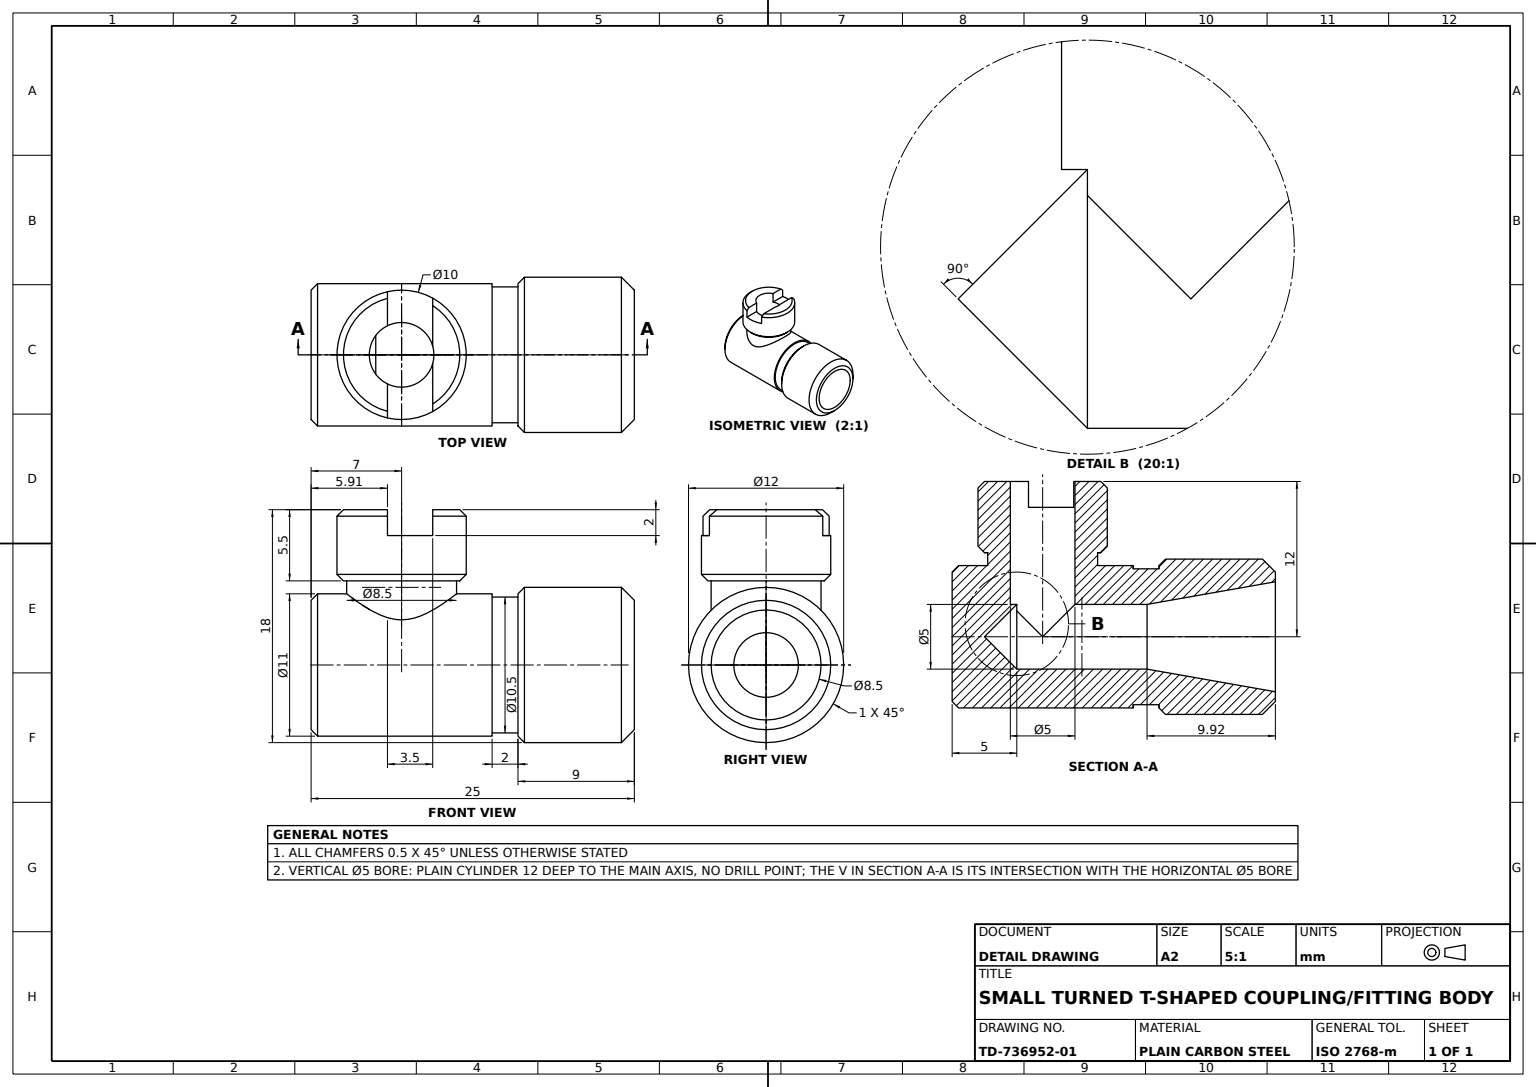
ISO-10303-21;
HEADER;
FILE_DESCRIPTION((''),'2;1');
FILE_NAME('','',(''),(''),'','','');
FILE_SCHEMA(('AUTOMOTIVE_DESIGN'));
ENDSEC;
DATA;
#1=APPLICATION_CONTEXT('');
#2=PRODUCT_CONTEXT('',#1,'mechanical');
#3=PRODUCT('','','',(#2));
#4=PRODUCT_DEFINITION_FORMATION('','',#3);
#5=PRODUCT_DEFINITION_CONTEXT('',#1,'design');
#6=PRODUCT_DEFINITION('','',#4,#5);
#7=PRODUCT_DEFINITION_SHAPE('','',#6);
#8=(LENGTH_UNIT()NAMED_UNIT(*)SI_UNIT(.MILLI.,.METRE.));
#9=(NAMED_UNIT(*)PLANE_ANGLE_UNIT()SI_UNIT($,.RADIAN.));
#10=(NAMED_UNIT(*)SI_UNIT($,.STERADIAN.)SOLID_ANGLE_UNIT());
#11=UNCERTAINTY_MEASURE_WITH_UNIT(LENGTH_MEASURE(1.E-05),#8,'distance_accuracy_value','');
#12=(GEOMETRIC_REPRESENTATION_CONTEXT(3)GLOBAL_UNCERTAINTY_ASSIGNED_CONTEXT((#11))GLOBAL_UNIT_ASSIGNED_CONTEXT((#8,#9,#10))REPRESENTATION_CONTEXT('',''));
#13=CARTESIAN_POINT('',(16.5,0.,6.));
#14=VERTEX_POINT('',#13);
#15=CARTESIAN_POINT('',(16.5,0.,-6.));
#16=VERTEX_POINT('',#15);
#17=CARTESIAN_POINT('',(16.5,0.,0.));
#18=DIRECTION('',(1.,0.,0.));
#19=DIRECTION('',(0.,0.,-1.));
#20=AXIS2_PLACEMENT_3D('',#17,#18,#19);
#21=CIRCLE('',#20,6.);
#22=EDGE_CURVE('',#14,#16,#21,.T.);
#23=ORIENTED_EDGE('',*,*,#22,.T.);
#24=CARTESIAN_POINT('',(24.,0.,-6.));
#25=VERTEX_POINT('',#24);
#26=CARTESIAN_POINT('',(-29.985577,0.,-6.));
#27=DIRECTION('',(-1.,0.,0.));
#28=VECTOR('',#27,1000.);
#29=LINE('',#26,#28);
#30=EDGE_CURVE('',#25,#16,#29,.T.);
#31=ORIENTED_EDGE('',*,*,#30,.F.);
#32=CARTESIAN_POINT('',(24.,0.,6.));
#33=VERTEX_POINT('',#32);
#34=CARTESIAN_POINT('',(24.,0.,0.));
#35=DIRECTION('',(0.,0.,1.));
#36=AXIS2_PLACEMENT_3D('',#34,#27,#35);
#37=CIRCLE('',#36,6.);
#38=EDGE_CURVE('',#25,#33,#37,.T.);
#39=ORIENTED_EDGE('',*,*,#38,.T.);
#40=CARTESIAN_POINT('',(-29.985577,0.,6.));
#41=LINE('',#40,#28);
#42=EDGE_CURVE('',#33,#14,#41,.T.);
#43=ORIENTED_EDGE('',*,*,#42,.T.);
#44=EDGE_LOOP('',(#23,#31,#39,#43));
#45=FACE_OUTER_BOUND('',#44,.T.);
#46=CARTESIAN_POINT('',(-29.985577,0.,0.));
#47=AXIS2_PLACEMENT_3D('',#46,#27,#35);
#48=CYLINDRICAL_SURFACE('',#47,6.);
#49=ADVANCED_FACE('',(#45),#48,.T.);
#50=CARTESIAN_POINT('',(16.,0.,-5.5));
#51=VERTEX_POINT('',#50);
#52=DIRECTION('',(0.707106781,0.,-0.707106781));
#53=VECTOR('',#52,1000.);
#54=LINE('',#50,#53);
#55=EDGE_CURVE('',#51,#16,#54,.T.);
#56=ORIENTED_EDGE('',*,*,#55,.T.);
#57=ORIENTED_EDGE('',*,*,#22,.F.);
#58=CARTESIAN_POINT('',(16.,0.,5.5));
#59=VERTEX_POINT('',#58);
#60=DIRECTION('',(0.707106781,0.,0.707106781));
#61=VECTOR('',#60,1000.);
#62=LINE('',#58,#61);
#63=EDGE_CURVE('',#59,#14,#62,.T.);
#64=ORIENTED_EDGE('',*,*,#63,.F.);
#65=CARTESIAN_POINT('',(16.,0.,0.));
#66=AXIS2_PLACEMENT_3D('',#65,#27,#19);
#67=CIRCLE('',#66,5.5);
#68=EDGE_CURVE('',#51,#59,#67,.T.);
#69=ORIENTED_EDGE('',*,*,#68,.F.);
#70=EDGE_LOOP('',(#56,#57,#64,#69));
#71=FACE_OUTER_BOUND('',#70,.T.);
#72=AXIS2_PLACEMENT_3D('',#65,#18,#19);
#73=CONICAL_SURFACE('',#72,5.5,0.785398163);
#74=ADVANCED_FACE('',(#71),#73,.T.);
#75=CARTESIAN_POINT('',(25.,0.,-5.));
#76=VERTEX_POINT('',#75);
#77=DIRECTION('',(-0.707106781,0.,-0.707106781));
#78=VECTOR('',#77,1000.);
#79=LINE('',#24,#78);
#80=EDGE_CURVE('',#76,#25,#79,.T.);
#81=ORIENTED_EDGE('',*,*,#80,.F.);
#82=CARTESIAN_POINT('',(25.,0.,5.));
#83=VERTEX_POINT('',#82);
#84=CARTESIAN_POINT('',(25.,0.,0.));
#85=AXIS2_PLACEMENT_3D('',#84,#18,#35);
#86=CIRCLE('',#85,5.);
#87=EDGE_CURVE('',#83,#76,#86,.T.);
#88=ORIENTED_EDGE('',*,*,#87,.F.);
#89=DIRECTION('',(-0.707106781,0.,0.707106781));
#90=VECTOR('',#89,1000.);
#91=LINE('',#32,#90);
#92=EDGE_CURVE('',#83,#33,#91,.T.);
#93=ORIENTED_EDGE('',*,*,#92,.T.);
#94=ORIENTED_EDGE('',*,*,#38,.F.);
#95=EDGE_LOOP('',(#81,#88,#93,#94));
#96=FACE_OUTER_BOUND('',#95,.T.);
#97=CONICAL_SURFACE('',#36,6.,0.785398163);
#98=ADVANCED_FACE('',(#96),#97,.T.);
#99=CARTESIAN_POINT('',(7.,6.5,4.5));
#100=VERTEX_POINT('',#99);
#101=CARTESIAN_POINT('',(7.,7.,5.));
#102=VERTEX_POINT('',#101);
#103=DIRECTION('',(0.,0.707106781,0.707106781));
#104=VECTOR('',#103,1000.);
#105=LINE('',#101,#104);
#106=EDGE_CURVE('',#100,#102,#105,.T.);
#107=ORIENTED_EDGE('',*,*,#106,.T.);
#108=CARTESIAN_POINT('',(7.,7.,-5.));
#109=VERTEX_POINT('',#108);
#110=CARTESIAN_POINT('',(7.,7.,0.));
#111=DIRECTION('',(0.,1.,0.));
#112=AXIS2_PLACEMENT_3D('',#110,#111,#35);
#113=CIRCLE('',#112,5.);
#114=EDGE_CURVE('',#109,#102,#113,.T.);
#115=ORIENTED_EDGE('',*,*,#114,.F.);
#116=CARTESIAN_POINT('',(7.,6.5,-4.5));
#117=VERTEX_POINT('',#116);
#118=DIRECTION('',(0.,0.707106781,-0.707106781));
#119=VECTOR('',#118,1000.);
#120=LINE('',#108,#119);
#121=EDGE_CURVE('',#117,#109,#120,.T.);
#122=ORIENTED_EDGE('',*,*,#121,.F.);
#123=CARTESIAN_POINT('',(7.,6.5,0.));
#124=DIRECTION('',(0.,-1.,0.));
#125=AXIS2_PLACEMENT_3D('',#123,#124,#35);
#126=CIRCLE('',#125,4.5);
#127=EDGE_CURVE('',#100,#117,#126,.T.);
#128=ORIENTED_EDGE('',*,*,#127,.F.);
#129=EDGE_LOOP('',(#107,#115,#122,#128));
#130=FACE_OUTER_BOUND('',#129,.T.);
#131=CONICAL_SURFACE('',#112,5.,0.785398163);
#132=ADVANCED_FACE('',(#130),#131,.T.);
#133=CARTESIAN_POINT('',(25.,0.,-4.25));
#134=VERTEX_POINT('',#133);
#135=CARTESIAN_POINT('',(25.,0.,4.25));
#136=VERTEX_POINT('',#135);
#137=AXIS2_PLACEMENT_3D('',#84,#27,#35);
#138=CIRCLE('',#137,4.25);
#139=EDGE_CURVE('',#134,#136,#138,.T.);
#140=ORIENTED_EDGE('',*,*,#139,.F.);
#141=CARTESIAN_POINT('',(15.075257,0.,-2.5));
#142=VERTEX_POINT('',#141);
#143=DIRECTION('',(0.984807753,0.,-0.173648178));
#144=VECTOR('',#143,1000.);
#145=LINE('',#133,#144);
#146=EDGE_CURVE('',#142,#134,#145,.T.);
#147=ORIENTED_EDGE('',*,*,#146,.F.);
#148=CARTESIAN_POINT('',(15.075257,0.,2.5));
#149=VERTEX_POINT('',#148);
#150=CARTESIAN_POINT('',(15.075257,0.,0.));
#151=AXIS2_PLACEMENT_3D('',#150,#27,#35);
#152=CIRCLE('',#151,2.5);
#153=EDGE_CURVE('',#142,#149,#152,.T.);
#154=ORIENTED_EDGE('',*,*,#153,.T.);
#155=DIRECTION('',(0.984807753,0.,0.173648178));
#156=VECTOR('',#155,1000.);
#157=LINE('',#135,#156);
#158=EDGE_CURVE('',#149,#136,#157,.T.);
#159=ORIENTED_EDGE('',*,*,#158,.T.);
#160=EDGE_LOOP('',(#140,#147,#154,#159));
#161=FACE_OUTER_BOUND('',#160,.T.);
#162=AXIS2_PLACEMENT_3D('',#84,#18,#19);
#163=CONICAL_SURFACE('',#162,4.25,0.174532925);
#164=ADVANCED_FACE('',(#161),#163,.F.);
#165=CARTESIAN_POINT('',(14.,0.,-5.5));
#166=VERTEX_POINT('',#165);
#167=CARTESIAN_POINT('',(0.5,0.,-5.5));
#168=VERTEX_POINT('',#167);
#169=CARTESIAN_POINT('',(-29.985577,0.,-5.5));
#170=LINE('',#169,#28);
#171=EDGE_CURVE('',#166,#168,#170,.T.);
#172=ORIENTED_EDGE('',*,*,#171,.T.);
#173=CARTESIAN_POINT('',(0.5,0.,5.5));
#174=VERTEX_POINT('',#173);
#175=CARTESIAN_POINT('',(0.5,0.,0.));
#176=AXIS2_PLACEMENT_3D('',#175,#18,#19);
#177=CIRCLE('',#176,5.5);
#178=EDGE_CURVE('',#168,#174,#177,.T.);
#179=ORIENTED_EDGE('',*,*,#178,.T.);
#180=CARTESIAN_POINT('',(14.,0.,5.5));
#181=VERTEX_POINT('',#180);
#182=CARTESIAN_POINT('',(-29.985577,0.,5.5));
#183=LINE('',#182,#28);
#184=EDGE_CURVE('',#181,#174,#183,.T.);
#185=ORIENTED_EDGE('',*,*,#184,.F.);
#186=CARTESIAN_POINT('',(14.,0.,0.));
#187=AXIS2_PLACEMENT_3D('',#186,#27,#35);
#188=CIRCLE('',#187,5.5);
#189=EDGE_CURVE('',#181,#166,#188,.T.);
#190=ORIENTED_EDGE('',*,*,#189,.T.);
#191=EDGE_LOOP('',(#172,#179,#185,#190));
#192=FACE_OUTER_BOUND('',#191,.T.);
#193=CARTESIAN_POINT('',(7.,3.49106,4.25));
#194=VERTEX_POINT('',#193);
#195=CARTESIAN_POINT('',(7.,3.49106,-4.25));
#196=VERTEX_POINT('',#195);
#197=CARTESIAN_POINT('',(7.297067,3.49106,4.25));
#198=CARTESIAN_POINT('',(7.583841,3.529202,4.219304));
#199=CARTESIAN_POINT('',(8.001594,3.629382,4.132739));
#200=CARTESIAN_POINT('',(8.13975,3.670262,4.096708));
#201=CARTESIAN_POINT('',(8.406532,3.761666,4.012943));
#202=CARTESIAN_POINT('',(8.535234,3.812052,3.965343));
#203=CARTESIAN_POINT('',(8.90971,3.972865,3.806449));
#204=CARTESIAN_POINT('',(9.144351,4.09292,3.67908));
#205=CARTESIAN_POINT('',(9.588183,4.34194,3.381595));
#206=CARTESIAN_POINT('',(9.792455,4.468184,3.214804));
#207=CARTESIAN_POINT('',(10.1703,4.713561,2.842881));
#208=CARTESIAN_POINT('',(10.345218,4.833854,2.635479));
#209=CARTESIAN_POINT('',(10.653427,5.052047,2.188312));
#210=CARTESIAN_POINT('',(10.787305,5.150302,1.948826));
#211=CARTESIAN_POINT('',(10.955145,5.275347,1.561763));
#212=CARTESIAN_POINT('',(11.005695,5.313406,1.427354));
#213=CARTESIAN_POINT('',(11.092546,5.379185,1.154988));
#214=CARTESIAN_POINT('',(11.129182,5.407151,1.016428));
#215=CARTESIAN_POINT('',(11.218236,5.475359,0.593348));
#216=CARTESIAN_POINT('',(11.249667,5.499743,0.29701));
#217=CARTESIAN_POINT('',(11.250327,5.500253,-0.287412));
#218=CARTESIAN_POINT('',(11.220652,5.477221,-0.577804));
#219=CARTESIAN_POINT('',(11.101971,5.386298,-1.149607));
#220=CARTESIAN_POINT('',(11.015304,5.320213,-1.420964));
#221=CARTESIAN_POINT('',(10.792714,5.154287,-1.938331));
#222=CARTESIAN_POINT('',(10.656887,5.054557,-2.182521));
#223=CARTESIAN_POINT('',(10.349426,4.836774,-2.630126));
#224=CARTESIAN_POINT('',(10.175044,4.716744,-2.837685));
#225=CARTESIAN_POINT('',(9.796141,4.470478,-3.211691));
#226=CARTESIAN_POINT('',(9.5922,4.344402,-3.378375));
#227=CARTESIAN_POINT('',(9.151826,4.096911,-3.674584));
#228=CARTESIAN_POINT('',(8.914007,3.974915,-3.804333));
#229=CARTESIAN_POINT('',(8.538855,3.813507,-3.963949));
#230=CARTESIAN_POINT('',(8.410286,3.763093,-4.011604));
#231=CARTESIAN_POINT('',(8.144787,3.671852,-4.095282));
#232=CARTESIAN_POINT('',(8.006834,3.630792,-4.131506));
#233=CARTESIAN_POINT('',(7.585708,3.529349,-4.219204));
#234=CARTESIAN_POINT('',(7.296083,3.49106,-4.25));
#235=B_SPLINE_CURVE_WITH_KNOTS('',3,(#193,#197,#198,#199,#200,#201,#202,#203,#204,#205,#206,#207,#208,#209,#210,#211,#212,#213,#214,#215,#216,#217,#218,#219,#220,#221,#222,#223,#224,#225,#226,#227,#228,#229,#230,#231,#232,#233,#234,#195),.UNSPECIFIED.,.F.,.F.,(4,2,2,2,2,2,2,2,2,2,2,2,2,2,2,2,2,2,2,4),(0.,0.000872118,0.001308177,0.001744236,0.002616354,0.003488473,0.004360591,0.005232709,0.005668768,0.006104827,0.006976945,0.007849063,0.008721182,0.0095933,0.010465418,0.011337536,0.012209654,0.012645713,0.013081772,0.013953891),.UNSPECIFIED.);
#236=EDGE_CURVE('',#194,#196,#235,.T.);
#237=ORIENTED_EDGE('',*,*,#236,.F.);
#238=CARTESIAN_POINT('',(6.703982,3.49106,-4.25));
#239=CARTESIAN_POINT('',(6.415826,3.529033,-4.219473));
#240=CARTESIAN_POINT('',(5.852708,3.664573,-4.102308));
#241=CARTESIAN_POINT('',(5.587933,3.75905,-4.017759));
#242=CARTESIAN_POINT('',(5.08781,3.97404,-3.80524));
#243=CARTESIAN_POINT('',(4.849817,4.096066,-3.67549));
#244=CARTESIAN_POINT('',(4.410515,4.342799,-3.380397));
#245=CARTESIAN_POINT('',(4.20721,4.468397,-3.214499));
#246=CARTESIAN_POINT('',(3.829638,4.713607,-2.842795));
#247=CARTESIAN_POINT('',(3.654452,4.834087,-2.635002));
#248=CARTESIAN_POINT('',(3.346898,5.051818,-2.188783));
#249=CARTESIAN_POINT('',(3.212841,5.150191,-1.94926));
#250=CARTESIAN_POINT('',(2.9883,5.317483,-1.431242));
#251=CARTESIAN_POINT('',(2.900545,5.384382,-1.157682));
#252=CARTESIAN_POINT('',(2.781688,5.475418,-0.592961));
#253=CARTESIAN_POINT('',(2.750315,5.499757,-0.296271));
#254=CARTESIAN_POINT('',(2.74969,5.500239,0.287178));
#255=CARTESIAN_POINT('',(2.779689,5.476958,0.579848));
#256=CARTESIAN_POINT('',(2.89817,5.386192,1.149885));
#257=CARTESIAN_POINT('',(2.984752,5.320167,1.421258));
#258=CARTESIAN_POINT('',(3.208004,5.153756,1.939834));
#259=CARTESIAN_POINT('',(3.343437,5.05432,2.183085));
#260=CARTESIAN_POINT('',(3.651174,4.836356,2.630908));
#261=CARTESIAN_POINT('',(3.825998,4.716047,2.838817));
#262=CARTESIAN_POINT('',(4.204506,4.470078,3.212225));
#263=CARTESIAN_POINT('',(4.408556,4.343929,3.379006));
#264=CARTESIAN_POINT('',(4.850122,4.095865,3.67577));
#265=CARTESIAN_POINT('',(5.087431,3.974227,3.805045));
#266=CARTESIAN_POINT('',(5.462412,3.812996,3.964438));
#267=CARTESIAN_POINT('',(5.591065,3.762577,4.012088));
#268=CARTESIAN_POINT('',(5.857128,3.671246,4.095826));
#269=CARTESIAN_POINT('',(5.995572,3.630141,4.132076));
#270=CARTESIAN_POINT('',(6.415387,3.52923,4.219294));
#271=CARTESIAN_POINT('',(6.702998,3.49106,4.25));
#272=B_SPLINE_CURVE_WITH_KNOTS('',3,(#195,#238,#239,#240,#241,#242,#243,#244,#245,#246,#247,#248,#249,#250,#251,#252,#253,#254,#255,#256,#257,#258,#259,#260,#261,#262,#263,#264,#265,#266,#267,#268,#269,#270,#271,#193),.UNSPECIFIED.,.F.,.F.,(4,2,2,2,2,2,2,2,2,2,2,2,2,2,2,2,2,4),(0.013953891,0.014825818,0.015697745,0.016569672,0.017441599,0.018313527,0.019185454,0.020057381,0.020929308,0.021801235,0.022673163,0.02354509,0.024417017,0.025288944,0.026160871,0.026596835,0.027032799,0.027904726),.UNSPECIFIED.);
#273=EDGE_CURVE('',#196,#194,#272,.T.);
#274=ORIENTED_EDGE('',*,*,#273,.F.);
#275=EDGE_LOOP('',(#237,#274));
#276=FACE_BOUND('',#275,.T.);
#277=CYLINDRICAL_SURFACE('',#47,5.5);
#278=ADVANCED_FACE('',(#192,#276),#277,.T.);
#279=ORIENTED_EDGE('',*,*,#92,.F.);
#280=EDGE_CURVE('',#76,#83,#86,.T.);
#281=ORIENTED_EDGE('',*,*,#280,.F.);
#282=ORIENTED_EDGE('',*,*,#80,.T.);
#283=EDGE_CURVE('',#33,#25,#37,.T.);
#284=ORIENTED_EDGE('',*,*,#283,.F.);
#285=EDGE_LOOP('',(#279,#281,#282,#284));
#286=FACE_OUTER_BOUND('',#285,.T.);
#287=ADVANCED_FACE('',(#286),#97,.T.);
#288=CARTESIAN_POINT('',(5.905319,10.,2.247593));
#289=VERTEX_POINT('',#288);
#290=CARTESIAN_POINT('',(5.905319,10.,4.878696));
#291=VERTEX_POINT('',#290);
#292=CARTESIAN_POINT('',(5.905319,10.,-7.75));
#293=VECTOR('',#35,1000.);
#294=LINE('',#292,#293);
#295=EDGE_CURVE('',#289,#291,#294,.T.);
#296=ORIENTED_EDGE('',*,*,#295,.F.);
#297=CARTESIAN_POINT('',(5.905319,12.,2.247593));
#298=VERTEX_POINT('',#297);
#299=CARTESIAN_POINT('',(5.905319,-6.001,2.247593));
#300=VECTOR('',#124,1000.);
#301=LINE('',#299,#300);
#302=EDGE_CURVE('',#298,#289,#301,.T.);
#303=ORIENTED_EDGE('',*,*,#302,.F.);
#304=CARTESIAN_POINT('',(5.905319,12.,4.364822));
#305=VERTEX_POINT('',#304);
#306=CARTESIAN_POINT('',(5.905319,12.,-7.75));
#307=LINE('',#306,#293);
#308=EDGE_CURVE('',#298,#305,#307,.T.);
#309=ORIENTED_EDGE('',*,*,#308,.T.);
#310=CARTESIAN_POINT('',(5.905319,11.5,4.878696));
#311=VERTEX_POINT('',#310);
#312=CARTESIAN_POINT('',(5.905319,11.833608,4.536368));
#313=CARTESIAN_POINT('',(5.905319,11.666913,4.707633));
#314=B_SPLINE_CURVE_WITH_KNOTS('',3,(#304,#312,#313,#310),.UNSPECIFIED.,.F.,.F.,(4,4),(0.011965922,0.01268712),.UNSPECIFIED.);
#315=EDGE_CURVE('',#305,#311,#314,.T.);
#316=ORIENTED_EDGE('',*,*,#315,.T.);
#317=CARTESIAN_POINT('',(5.905319,6.5,4.878696));
#318=LINE('',#317,#300);
#319=EDGE_CURVE('',#311,#291,#318,.T.);
#320=ORIENTED_EDGE('',*,*,#319,.T.);
#321=EDGE_LOOP('',(#296,#303,#309,#316,#320));
#322=FACE_OUTER_BOUND('',#321,.T.);
#323=AXIS2_PLACEMENT_3D('',#306,#27,#35);
#324=PLANE('',#323);
#325=ADVANCED_FACE('',(#322),#324,.F.);
#326=CARTESIAN_POINT('',(16.,0.,5.25));
#327=VERTEX_POINT('',#326);
#328=CARTESIAN_POINT('',(14.,0.,5.25));
#329=VERTEX_POINT('',#328);
#330=CARTESIAN_POINT('',(-29.985577,0.,5.25));
#331=LINE('',#330,#28);
#332=EDGE_CURVE('',#327,#329,#331,.T.);
#333=ORIENTED_EDGE('',*,*,#332,.T.);
#334=CARTESIAN_POINT('',(14.,0.,-5.25));
#335=VERTEX_POINT('',#334);
#336=CIRCLE('',#187,5.25);
#337=EDGE_CURVE('',#335,#329,#336,.T.);
#338=ORIENTED_EDGE('',*,*,#337,.F.);
#339=CARTESIAN_POINT('',(16.,0.,-5.25));
#340=VERTEX_POINT('',#339);
#341=CARTESIAN_POINT('',(-29.985577,0.,-5.25));
#342=LINE('',#341,#28);
#343=EDGE_CURVE('',#340,#335,#342,.T.);
#344=ORIENTED_EDGE('',*,*,#343,.F.);
#345=AXIS2_PLACEMENT_3D('',#65,#27,#35);
#346=CIRCLE('',#345,5.25);
#347=EDGE_CURVE('',#340,#327,#346,.T.);
#348=ORIENTED_EDGE('',*,*,#347,.T.);
#349=EDGE_LOOP('',(#333,#338,#344,#348));
#350=FACE_OUTER_BOUND('',#349,.T.);
#351=CYLINDRICAL_SURFACE('',#47,5.25);
#352=ADVANCED_FACE('',(#350),#351,.T.);
#353=CARTESIAN_POINT('',(7.,10.,5.));
#354=VERTEX_POINT('',#353);
#355=CARTESIAN_POINT('',(7.,10.,0.));
#356=AXIS2_PLACEMENT_3D('',#355,#111,#19);
#357=CIRCLE('',#356,5.);
#358=EDGE_CURVE('',#291,#354,#357,.T.);
#359=ORIENTED_EDGE('',*,*,#358,.T.);
#360=CARTESIAN_POINT('',(9.405319,10.,4.383428));
#361=VERTEX_POINT('',#360);
#362=EDGE_CURVE('',#354,#361,#357,.T.);
#363=ORIENTED_EDGE('',*,*,#362,.T.);
#364=CARTESIAN_POINT('',(9.405319,10.,0.6815));
#365=VERTEX_POINT('',#364);
#366=CARTESIAN_POINT('',(9.405319,10.,-7.75));
#367=LINE('',#366,#293);
#368=EDGE_CURVE('',#365,#361,#367,.T.);
#369=ORIENTED_EDGE('',*,*,#368,.F.);
#370=CARTESIAN_POINT('',(7.,10.,2.5));
#371=VERTEX_POINT('',#370);
#372=CIRCLE('',#356,2.5);
#373=EDGE_CURVE('',#371,#365,#372,.T.);
#374=ORIENTED_EDGE('',*,*,#373,.F.);
#375=EDGE_CURVE('',#289,#371,#372,.T.);
#376=ORIENTED_EDGE('',*,*,#375,.F.);
#377=ORIENTED_EDGE('',*,*,#295,.T.);
#378=EDGE_LOOP('',(#359,#363,#369,#374,#376,#377));
#379=FACE_OUTER_BOUND('',#378,.T.);
#380=AXIS2_PLACEMENT_3D('',#292,#124,#19);
#381=PLANE('',#380);
#382=ADVANCED_FACE('',(#379),#381,.F.);
#383=CARTESIAN_POINT('',(5.,2.,-1.5));
#384=VERTEX_POINT('',#383);
#385=CARTESIAN_POINT('',(5.,0.,-2.5));
#386=VERTEX_POINT('',#385);
#387=CARTESIAN_POINT('',(5.,0.,0.));
#388=AXIS2_PLACEMENT_3D('',#387,#27,#35);
#389=CIRCLE('',#388,2.5);
#390=EDGE_CURVE('',#384,#386,#389,.T.);
#391=ORIENTED_EDGE('',*,*,#390,.F.);
#392=CARTESIAN_POINT('',(5.,2.,1.5));
#393=VERTEX_POINT('',#392);
#394=EDGE_CURVE('',#393,#384,#389,.T.);
#395=ORIENTED_EDGE('',*,*,#394,.F.);
#396=CARTESIAN_POINT('',(5.,0.,2.5));
#397=VERTEX_POINT('',#396);
#398=EDGE_CURVE('',#397,#393,#389,.T.);
#399=ORIENTED_EDGE('',*,*,#398,.F.);
#400=CARTESIAN_POINT('',(2.5,0.,0.));
#401=VERTEX_POINT('',#400);
#402=LINE('',#396,#61);
#403=EDGE_CURVE('',#401,#397,#402,.T.);
#404=ORIENTED_EDGE('',*,*,#403,.F.);
#405=LINE('',#385,#53);
#406=EDGE_CURVE('',#401,#386,#405,.T.);
#407=ORIENTED_EDGE('',*,*,#406,.T.);
#408=EDGE_LOOP('',(#391,#395,#399,#404,#407));
#409=FACE_OUTER_BOUND('',#408,.T.);
#410=AXIS2_PLACEMENT_3D('',#387,#18,#19);
#411=CONICAL_SURFACE('',#410,2.5,0.785398163);
#412=ADVANCED_FACE('',(#409),#411,.F.);
#413=EDGE_CURVE('',#166,#181,#188,.T.);
#414=ORIENTED_EDGE('',*,*,#413,.T.);
#415=ORIENTED_EDGE('',*,*,#184,.T.);
#416=EDGE_CURVE('',#174,#168,#177,.T.);
#417=ORIENTED_EDGE('',*,*,#416,.T.);
#418=ORIENTED_EDGE('',*,*,#171,.F.);
#419=EDGE_LOOP('',(#414,#415,#417,#418));
#420=FACE_OUTER_BOUND('',#419,.T.);
#421=ADVANCED_FACE('',(#420),#277,.T.);
#422=EDGE_CURVE('',#117,#100,#126,.T.);
#423=ORIENTED_EDGE('',*,*,#422,.F.);
#424=ORIENTED_EDGE('',*,*,#121,.T.);
#425=EDGE_CURVE('',#102,#109,#113,.T.);
#426=ORIENTED_EDGE('',*,*,#425,.F.);
#427=ORIENTED_EDGE('',*,*,#106,.F.);
#428=EDGE_LOOP('',(#423,#424,#426,#427));
#429=FACE_OUTER_BOUND('',#428,.T.);
#430=ADVANCED_FACE('',(#429),#131,.T.);
#431=ORIENTED_EDGE('',*,*,#63,.T.);
#432=EDGE_CURVE('',#16,#14,#21,.T.);
#433=ORIENTED_EDGE('',*,*,#432,.F.);
#434=ORIENTED_EDGE('',*,*,#55,.F.);
#435=EDGE_CURVE('',#59,#51,#67,.T.);
#436=ORIENTED_EDGE('',*,*,#435,.F.);
#437=EDGE_LOOP('',(#431,#433,#434,#436));
#438=FACE_OUTER_BOUND('',#437,.T.);
#439=ADVANCED_FACE('',(#438),#73,.T.);
#440=ORIENTED_EDGE('',*,*,#368,.T.);
#441=CARTESIAN_POINT('',(9.405319,11.5,4.383428));
#442=VERTEX_POINT('',#441);
#443=CARTESIAN_POINT('',(9.405319,6.5,4.383428));
#444=VECTOR('',#111,1000.);
#445=LINE('',#443,#444);
#446=EDGE_CURVE('',#361,#442,#445,.T.);
#447=ORIENTED_EDGE('',*,*,#446,.T.);
#448=CARTESIAN_POINT('',(9.405319,12.,3.803215));
#449=VERTEX_POINT('',#448);
#450=CARTESIAN_POINT('',(9.405319,11.668342,4.191407));
#451=CARTESIAN_POINT('',(9.405319,11.835223,3.99818));
#452=B_SPLINE_CURVE_WITH_KNOTS('',3,(#441,#450,#451,#448),.UNSPECIFIED.,.F.,.F.,(4,4),(0.000001061,0.000766823),.UNSPECIFIED.);
#453=EDGE_CURVE('',#442,#449,#452,.T.);
#454=ORIENTED_EDGE('',*,*,#453,.T.);
#455=CARTESIAN_POINT('',(9.405319,12.,0.6815));
#456=VERTEX_POINT('',#455);
#457=CARTESIAN_POINT('',(9.405319,12.,-7.75));
#458=LINE('',#457,#293);
#459=EDGE_CURVE('',#456,#449,#458,.T.);
#460=ORIENTED_EDGE('',*,*,#459,.F.);
#461=CARTESIAN_POINT('',(9.405319,-6.001,0.6815));
#462=LINE('',#461,#444);
#463=EDGE_CURVE('',#365,#456,#462,.T.);
#464=ORIENTED_EDGE('',*,*,#463,.F.);
#465=EDGE_LOOP('',(#440,#447,#454,#460,#464));
#466=FACE_OUTER_BOUND('',#465,.T.);
#467=AXIS2_PLACEMENT_3D('',#366,#18,#19);
#468=PLANE('',#467);
#469=ADVANCED_FACE('',(#466),#468,.F.);
#470=ORIENTED_EDGE('',*,*,#403,.T.);
#471=EDGE_CURVE('',#386,#397,#389,.T.);
#472=ORIENTED_EDGE('',*,*,#471,.F.);
#473=ORIENTED_EDGE('',*,*,#406,.F.);
#474=EDGE_LOOP('',(#470,#472,#473));
#475=FACE_OUTER_BOUND('',#474,.T.);
#476=ADVANCED_FACE('',(#475),#411,.F.);
#477=ORIENTED_EDGE('',*,*,#315,.F.);
#478=CARTESIAN_POINT('',(5.905319,12.,-4.364822));
#479=VERTEX_POINT('',#478);
#480=CARTESIAN_POINT('',(7.,12.,0.));
#481=AXIS2_PLACEMENT_3D('',#480,#111,#35);
#482=CIRCLE('',#481,4.5);
#483=EDGE_CURVE('',#479,#305,#482,.T.);
#484=ORIENTED_EDGE('',*,*,#483,.F.);
#485=CARTESIAN_POINT('',(5.905319,11.5,-4.878696));
#486=VERTEX_POINT('',#485);
#487=CARTESIAN_POINT('',(5.905319,11.666913,-4.707633));
#488=CARTESIAN_POINT('',(5.905319,11.833608,-4.536368));
#489=B_SPLINE_CURVE_WITH_KNOTS('',3,(#485,#487,#488,#478),.UNSPECIFIED.,.F.,.F.,(4,4),(0.000001002,0.000717781),.UNSPECIFIED.);
#490=EDGE_CURVE('',#486,#479,#489,.T.);
#491=ORIENTED_EDGE('',*,*,#490,.F.);
#492=CARTESIAN_POINT('',(7.,11.5,0.));
#493=AXIS2_PLACEMENT_3D('',#492,#124,#35);
#494=CIRCLE('',#493,5.);
#495=EDGE_CURVE('',#311,#486,#494,.T.);
#496=ORIENTED_EDGE('',*,*,#495,.F.);
#497=EDGE_LOOP('',(#477,#484,#491,#496));
#498=FACE_OUTER_BOUND('',#497,.T.);
#499=AXIS2_PLACEMENT_3D('',#480,#124,#19);
#500=CONICAL_SURFACE('',#499,4.5,0.785398163);
#501=ADVANCED_FACE('',(#498),#500,.T.);
#502=ORIENTED_EDGE('',*,*,#189,.F.);
#503=ORIENTED_EDGE('',*,*,#413,.F.);
#504=EDGE_LOOP('',(#502,#503));
#505=FACE_OUTER_BOUND('',#504,.T.);
#506=EDGE_CURVE('',#329,#335,#336,.T.);
#507=ORIENTED_EDGE('',*,*,#506,.T.);
#508=ORIENTED_EDGE('',*,*,#337,.T.);
#509=EDGE_LOOP('',(#507,#508));
#510=FACE_BOUND('',#509,.T.);
#511=CARTESIAN_POINT('',(14.,5.5,0.));
#512=AXIS2_PLACEMENT_3D('',#511,#27,#35);
#513=PLANE('',#512);
#514=ADVANCED_FACE('',(#505,#510),#513,.F.);
#515=ORIENTED_EDGE('',*,*,#432,.T.);
#516=ORIENTED_EDGE('',*,*,#42,.F.);
#517=ORIENTED_EDGE('',*,*,#283,.T.);
#518=ORIENTED_EDGE('',*,*,#30,.T.);
#519=EDGE_LOOP('',(#515,#516,#517,#518));
#520=FACE_OUTER_BOUND('',#519,.T.);
#521=ADVANCED_FACE('',(#520),#48,.T.);
#522=CARTESIAN_POINT('',(7.,6.5,4.25));
#523=VERTEX_POINT('',#522);
#524=CARTESIAN_POINT('',(7.,-6.001,4.25));
#525=LINE('',#524,#444);
#526=EDGE_CURVE('',#194,#523,#525,.T.);
#527=ORIENTED_EDGE('',*,*,#526,.T.);
#528=CARTESIAN_POINT('',(7.,6.5,-4.25));
#529=VERTEX_POINT('',#528);
#530=AXIS2_PLACEMENT_3D('',#123,#124,#19);
#531=CIRCLE('',#530,4.25);
#532=EDGE_CURVE('',#523,#529,#531,.T.);
#533=ORIENTED_EDGE('',*,*,#532,.T.);
#534=CARTESIAN_POINT('',(7.,-6.001,-4.25));
#535=LINE('',#534,#444);
#536=EDGE_CURVE('',#196,#529,#535,.T.);
#537=ORIENTED_EDGE('',*,*,#536,.F.);
#538=ORIENTED_EDGE('',*,*,#273,.T.);
#539=EDGE_LOOP('',(#527,#533,#537,#538));
#540=FACE_OUTER_BOUND('',#539,.T.);
#541=CARTESIAN_POINT('',(7.,-6.001,0.));
#542=AXIS2_PLACEMENT_3D('',#541,#111,#35);
#543=CYLINDRICAL_SURFACE('',#542,4.25);
#544=ADVANCED_FACE('',(#540),#543,.T.);
#545=CARTESIAN_POINT('',(4.307692,2.692308,-0.576923));
#546=CARTESIAN_POINT('',(4.307692,2.692308,0.576923));
#547=(BOUNDED_CURVE()B_SPLINE_CURVE(3,(#383,#545,#546,#392),.UNSPECIFIED.,.F.,.T.)B_SPLINE_CURVE_WITH_KNOTS((4,4),(5.639684198,6.926686416),.UNSPECIFIED.)CURVE()GEOMETRIC_REPRESENTATION_ITEM()RATIONAL_B_SPLINE_CURVE((1.,0.866666667,0.866666667,1.))REPRESENTATION_ITEM(''));
#548=EDGE_CURVE('',#384,#393,#547,.T.);
#549=ORIENTED_EDGE('',*,*,#548,.T.);
#550=ORIENTED_EDGE('',*,*,#394,.T.);
#551=EDGE_LOOP('',(#549,#550));
#552=FACE_OUTER_BOUND('',#551,.T.);
#553=CARTESIAN_POINT('',(0.,0.,0.));
#554=AXIS2_PLACEMENT_3D('',#553,#27,#35);
#555=CYLINDRICAL_SURFACE('',#554,2.5);
#556=ADVANCED_FACE('',(#552),#555,.T.);
#557=CARTESIAN_POINT('',(5.905319,10.,-2.247593));
#558=VERTEX_POINT('',#557);
#559=CARTESIAN_POINT('',(5.905319,12.,-2.247593));
#560=VERTEX_POINT('',#559);
#561=CARTESIAN_POINT('',(5.905319,-6.001,-2.247593));
#562=LINE('',#561,#444);
#563=EDGE_CURVE('',#558,#560,#562,.T.);
#564=ORIENTED_EDGE('',*,*,#563,.F.);
#565=CARTESIAN_POINT('',(5.905319,10.,-4.878696));
#566=VERTEX_POINT('',#565);
#567=EDGE_CURVE('',#566,#558,#294,.T.);
#568=ORIENTED_EDGE('',*,*,#567,.F.);
#569=CARTESIAN_POINT('',(5.905319,6.5,-4.878696));
#570=LINE('',#569,#444);
#571=EDGE_CURVE('',#566,#486,#570,.T.);
#572=ORIENTED_EDGE('',*,*,#571,.T.);
#573=ORIENTED_EDGE('',*,*,#490,.T.);
#574=EDGE_CURVE('',#479,#560,#307,.T.);
#575=ORIENTED_EDGE('',*,*,#574,.T.);
#576=EDGE_LOOP('',(#564,#568,#572,#573,#575));
#577=FACE_OUTER_BOUND('',#576,.T.);
#578=ADVANCED_FACE('',(#577),#324,.F.);
#579=CARTESIAN_POINT('',(7.,0.,-2.5));
#580=VERTEX_POINT('',#579);
#581=CARTESIAN_POINT('',(0.,0.,-2.5));
#582=LINE('',#581,#28);
#583=EDGE_CURVE('',#580,#386,#582,.T.);
#584=ORIENTED_EDGE('',*,*,#583,.F.);
#585=CARTESIAN_POINT('',(6.198213,0.801787,-2.5));
#586=CARTESIAN_POINT('',(5.481072,1.518928,-2.14143));
#587=(BOUNDED_CURVE()B_SPLINE_CURVE(3,(#579,#585,#586,#383),.UNSPECIFIED.,.F.,.T.)B_SPLINE_CURVE_WITH_KNOTS((4,4),(4.71238898,5.639684198),.UNSPECIFIED.)CURVE()GEOMETRIC_REPRESENTATION_ITEM()RATIONAL_B_SPLINE_CURVE((1.,0.929618127,0.929618127,1.))REPRESENTATION_ITEM(''));
#588=EDGE_CURVE('',#580,#384,#587,.T.);
#589=ORIENTED_EDGE('',*,*,#588,.T.);
#590=ORIENTED_EDGE('',*,*,#390,.T.);
#591=EDGE_LOOP('',(#584,#589,#590));
#592=FACE_OUTER_BOUND('',#591,.T.);
#593=ADVANCED_FACE('',(#592),#555,.F.);
#594=ORIENTED_EDGE('',*,*,#416,.F.);
#595=CARTESIAN_POINT('',(0.,0.,5.));
#596=VERTEX_POINT('',#595);
#597=LINE('',#595,#61);
#598=EDGE_CURVE('',#596,#174,#597,.T.);
#599=ORIENTED_EDGE('',*,*,#598,.F.);
#600=CARTESIAN_POINT('',(0.,0.,-5.));
#601=VERTEX_POINT('',#600);
#602=AXIS2_PLACEMENT_3D('',#553,#27,#19);
#603=CIRCLE('',#602,5.);
#604=EDGE_CURVE('',#601,#596,#603,.T.);
#605=ORIENTED_EDGE('',*,*,#604,.F.);
#606=LINE('',#600,#53);
#607=EDGE_CURVE('',#601,#168,#606,.T.);
#608=ORIENTED_EDGE('',*,*,#607,.T.);
#609=EDGE_LOOP('',(#594,#599,#605,#608));
#610=FACE_OUTER_BOUND('',#609,.T.);
#611=AXIS2_PLACEMENT_3D('',#553,#18,#19);
#612=CONICAL_SURFACE('',#611,5.,0.785398163);
#613=ADVANCED_FACE('',(#610),#612,.T.);
#614=CARTESIAN_POINT('',(7.,10.,-5.));
#615=VERTEX_POINT('',#614);
#616=CARTESIAN_POINT('',(7.,6.5,-5.));
#617=LINE('',#616,#444);
#618=EDGE_CURVE('',#109,#615,#617,.T.);
#619=ORIENTED_EDGE('',*,*,#618,.F.);
#620=ORIENTED_EDGE('',*,*,#114,.T.);
#621=CARTESIAN_POINT('',(7.,6.5,5.));
#622=LINE('',#621,#444);
#623=EDGE_CURVE('',#102,#354,#622,.T.);
#624=ORIENTED_EDGE('',*,*,#623,.T.);
#625=ORIENTED_EDGE('',*,*,#358,.F.);
#626=ORIENTED_EDGE('',*,*,#319,.F.);
#627=ORIENTED_EDGE('',*,*,#495,.T.);
#628=ORIENTED_EDGE('',*,*,#571,.F.);
#629=EDGE_CURVE('',#615,#566,#357,.T.);
#630=ORIENTED_EDGE('',*,*,#629,.F.);
#631=EDGE_LOOP('',(#619,#620,#624,#625,#626,#627,#628,#630));
#632=FACE_OUTER_BOUND('',#631,.T.);
#633=AXIS2_PLACEMENT_3D('',#123,#111,#35);
#634=CYLINDRICAL_SURFACE('',#633,5.);
#635=ADVANCED_FACE('',(#632),#634,.T.);
#636=CARTESIAN_POINT('',(9.405319,11.5,-4.383428));
#637=VERTEX_POINT('',#636);
#638=EDGE_CURVE('',#637,#442,#494,.T.);
#639=ORIENTED_EDGE('',*,*,#638,.F.);
#640=CARTESIAN_POINT('',(9.405319,12.,-3.803215));
#641=VERTEX_POINT('',#640);
#642=CARTESIAN_POINT('',(9.405319,11.835209,-3.998197));
#643=CARTESIAN_POINT('',(9.405319,11.668329,-4.191422));
#644=B_SPLINE_CURVE_WITH_KNOTS('',3,(#640,#642,#643,#636),.UNSPECIFIED.,.F.,.F.,(4,4),(0.0096229,0.010390024),.UNSPECIFIED.);
#645=EDGE_CURVE('',#641,#637,#644,.T.);
#646=ORIENTED_EDGE('',*,*,#645,.F.);
#647=EDGE_CURVE('',#449,#641,#482,.T.);
#648=ORIENTED_EDGE('',*,*,#647,.F.);
#649=ORIENTED_EDGE('',*,*,#453,.F.);
#650=EDGE_LOOP('',(#639,#646,#648,#649));
#651=FACE_OUTER_BOUND('',#650,.T.);
#652=ADVANCED_FACE('',(#651),#500,.T.);
#653=ORIENTED_EDGE('',*,*,#645,.T.);
#654=CARTESIAN_POINT('',(9.405319,10.,-4.383428));
#655=VERTEX_POINT('',#654);
#656=CARTESIAN_POINT('',(9.405319,6.5,-4.383428));
#657=LINE('',#656,#300);
#658=EDGE_CURVE('',#637,#655,#657,.T.);
#659=ORIENTED_EDGE('',*,*,#658,.T.);
#660=CARTESIAN_POINT('',(9.405319,10.,-0.6815));
#661=VERTEX_POINT('',#660);
#662=EDGE_CURVE('',#655,#661,#367,.T.);
#663=ORIENTED_EDGE('',*,*,#662,.T.);
#664=CARTESIAN_POINT('',(9.405319,12.,-0.6815));
#665=VERTEX_POINT('',#664);
#666=CARTESIAN_POINT('',(9.405319,-6.001,-0.6815));
#667=LINE('',#666,#300);
#668=EDGE_CURVE('',#665,#661,#667,.T.);
#669=ORIENTED_EDGE('',*,*,#668,.F.);
#670=EDGE_CURVE('',#641,#665,#458,.T.);
#671=ORIENTED_EDGE('',*,*,#670,.F.);
#672=EDGE_LOOP('',(#653,#659,#663,#669,#671));
#673=FACE_OUTER_BOUND('',#672,.T.);
#674=ADVANCED_FACE('',(#673),#468,.F.);
#675=ORIENTED_EDGE('',*,*,#588,.F.);
#676=CARTESIAN_POINT('',(7.,10.,-2.5));
#677=VERTEX_POINT('',#676);
#678=CARTESIAN_POINT('',(7.,-6.001,-2.5));
#679=LINE('',#678,#444);
#680=EDGE_CURVE('',#580,#677,#679,.T.);
#681=ORIENTED_EDGE('',*,*,#680,.T.);
#682=EDGE_CURVE('',#677,#558,#372,.T.);
#683=ORIENTED_EDGE('',*,*,#682,.T.);
#684=ORIENTED_EDGE('',*,*,#563,.T.);
#685=CIRCLE('',#481,2.5);
#686=EDGE_CURVE('',#560,#298,#685,.T.);
#687=ORIENTED_EDGE('',*,*,#686,.T.);
#688=ORIENTED_EDGE('',*,*,#302,.T.);
#689=ORIENTED_EDGE('',*,*,#375,.T.);
#690=CARTESIAN_POINT('',(7.,0.,2.5));
#691=VERTEX_POINT('',#690);
#692=CARTESIAN_POINT('',(7.,-6.001,2.5));
#693=LINE('',#692,#444);
#694=EDGE_CURVE('',#691,#371,#693,.T.);
#695=ORIENTED_EDGE('',*,*,#694,.F.);
#696=CARTESIAN_POINT('',(5.481072,1.518928,2.14143));
#697=CARTESIAN_POINT('',(6.198213,0.801787,2.5));
#698=(BOUNDED_CURVE()B_SPLINE_CURVE(3,(#392,#696,#697,#690),.UNSPECIFIED.,.F.,.T.)B_SPLINE_CURVE_WITH_KNOTS((4,4),(0.643501109,1.570796327),.UNSPECIFIED.)CURVE()GEOMETRIC_REPRESENTATION_ITEM()RATIONAL_B_SPLINE_CURVE((1.,0.929618127,0.929618127,1.))REPRESENTATION_ITEM(''));
#699=EDGE_CURVE('',#393,#691,#698,.T.);
#700=ORIENTED_EDGE('',*,*,#699,.F.);
#701=ORIENTED_EDGE('',*,*,#548,.F.);
#702=EDGE_LOOP('',(#675,#681,#683,#684,#687,#688,#689,#695,#700,#701));
#703=FACE_OUTER_BOUND('',#702,.T.);
#704=CYLINDRICAL_SURFACE('',#542,2.5);
#705=ADVANCED_FACE('',(#703),#704,.F.);
#706=ORIENTED_EDGE('',*,*,#536,.T.);
#707=EDGE_CURVE('',#529,#523,#531,.T.);
#708=ORIENTED_EDGE('',*,*,#707,.T.);
#709=ORIENTED_EDGE('',*,*,#526,.F.);
#710=ORIENTED_EDGE('',*,*,#236,.T.);
#711=EDGE_LOOP('',(#706,#708,#709,#710));
#712=FACE_OUTER_BOUND('',#711,.T.);
#713=ADVANCED_FACE('',(#712),#543,.T.);
#714=CARTESIAN_POINT('',(0.,0.,2.5));
#715=LINE('',#714,#28);
#716=EDGE_CURVE('',#149,#691,#715,.T.);
#717=ORIENTED_EDGE('',*,*,#716,.F.);
#718=ORIENTED_EDGE('',*,*,#153,.F.);
#719=EDGE_CURVE('',#142,#580,#582,.T.);
#720=ORIENTED_EDGE('',*,*,#719,.T.);
#721=ORIENTED_EDGE('',*,*,#583,.T.);
#722=ORIENTED_EDGE('',*,*,#471,.T.);
#723=EDGE_CURVE('',#691,#397,#715,.T.);
#724=ORIENTED_EDGE('',*,*,#723,.F.);
#725=EDGE_LOOP('',(#717,#718,#720,#721,#722,#724));
#726=FACE_OUTER_BOUND('',#725,.T.);
#727=ADVANCED_FACE('',(#726),#555,.F.);
#728=ORIENTED_EDGE('',*,*,#373,.T.);
#729=ORIENTED_EDGE('',*,*,#463,.T.);
#730=EDGE_CURVE('',#456,#665,#685,.T.);
#731=ORIENTED_EDGE('',*,*,#730,.T.);
#732=ORIENTED_EDGE('',*,*,#668,.T.);
#733=EDGE_CURVE('',#661,#677,#372,.T.);
#734=ORIENTED_EDGE('',*,*,#733,.T.);
#735=ORIENTED_EDGE('',*,*,#680,.F.);
#736=CARTESIAN_POINT('',(12.,5.,2.5));
#737=CARTESIAN_POINT('',(12.,5.,-2.5));
#738=(BOUNDED_CURVE()B_SPLINE_CURVE(3,(#690,#736,#737,#579),.UNSPECIFIED.,.F.,.T.)B_SPLINE_CURVE_WITH_KNOTS((4,4),(4.71238898,7.853981634),.UNSPECIFIED.)CURVE()GEOMETRIC_REPRESENTATION_ITEM()RATIONAL_B_SPLINE_CURVE((1.,0.333333333,0.333333333,1.))REPRESENTATION_ITEM(''));
#739=EDGE_CURVE('',#691,#580,#738,.T.);
#740=ORIENTED_EDGE('',*,*,#739,.F.);
#741=ORIENTED_EDGE('',*,*,#694,.T.);
#742=EDGE_LOOP('',(#728,#729,#731,#732,#734,#735,#740,#741));
#743=FACE_OUTER_BOUND('',#742,.T.);
#744=ADVANCED_FACE('',(#743),#704,.F.);
#745=EDGE_CURVE('',#136,#134,#138,.T.);
#746=ORIENTED_EDGE('',*,*,#745,.T.);
#747=ORIENTED_EDGE('',*,*,#139,.T.);
#748=EDGE_LOOP('',(#746,#747));
#749=FACE_BOUND('',#748,.T.);
#750=ORIENTED_EDGE('',*,*,#87,.T.);
#751=ORIENTED_EDGE('',*,*,#280,.T.);
#752=EDGE_LOOP('',(#750,#751));
#753=FACE_OUTER_BOUND('',#752,.T.);
#754=CARTESIAN_POINT('',(25.,6.,0.));
#755=AXIS2_PLACEMENT_3D('',#754,#27,#35);
#756=PLANE('',#755);
#757=ADVANCED_FACE('',(#749,#753),#756,.F.);
#758=ORIENTED_EDGE('',*,*,#739,.T.);
#759=ORIENTED_EDGE('',*,*,#719,.F.);
#760=EDGE_CURVE('',#149,#142,#152,.T.);
#761=ORIENTED_EDGE('',*,*,#760,.F.);
#762=ORIENTED_EDGE('',*,*,#716,.T.);
#763=EDGE_LOOP('',(#758,#759,#761,#762));
#764=FACE_OUTER_BOUND('',#763,.T.);
#765=ADVANCED_FACE('',(#764),#555,.F.);
#766=EDGE_CURVE('',#327,#340,#346,.T.);
#767=ORIENTED_EDGE('',*,*,#766,.T.);
#768=ORIENTED_EDGE('',*,*,#343,.T.);
#769=ORIENTED_EDGE('',*,*,#506,.F.);
#770=ORIENTED_EDGE('',*,*,#332,.F.);
#771=EDGE_LOOP('',(#767,#768,#769,#770));
#772=FACE_OUTER_BOUND('',#771,.T.);
#773=ADVANCED_FACE('',(#772),#351,.T.);
#774=ORIENTED_EDGE('',*,*,#670,.T.);
#775=ORIENTED_EDGE('',*,*,#730,.F.);
#776=ORIENTED_EDGE('',*,*,#459,.T.);
#777=ORIENTED_EDGE('',*,*,#647,.T.);
#778=EDGE_LOOP('',(#774,#775,#776,#777));
#779=FACE_OUTER_BOUND('',#778,.T.);
#780=PLANE('',#481);
#781=ADVANCED_FACE('',(#779),#780,.T.);
#782=ORIENTED_EDGE('',*,*,#618,.T.);
#783=EDGE_CURVE('',#655,#615,#357,.T.);
#784=ORIENTED_EDGE('',*,*,#783,.F.);
#785=ORIENTED_EDGE('',*,*,#658,.F.);
#786=ORIENTED_EDGE('',*,*,#638,.T.);
#787=ORIENTED_EDGE('',*,*,#446,.F.);
#788=ORIENTED_EDGE('',*,*,#362,.F.);
#789=ORIENTED_EDGE('',*,*,#623,.F.);
#790=ORIENTED_EDGE('',*,*,#425,.T.);
#791=EDGE_LOOP('',(#782,#784,#785,#786,#787,#788,#789,#790));
#792=FACE_OUTER_BOUND('',#791,.T.);
#793=ADVANCED_FACE('',(#792),#634,.T.);
#794=ORIENTED_EDGE('',*,*,#347,.F.);
#795=ORIENTED_EDGE('',*,*,#766,.F.);
#796=EDGE_LOOP('',(#794,#795));
#797=FACE_BOUND('',#796,.T.);
#798=ORIENTED_EDGE('',*,*,#435,.T.);
#799=ORIENTED_EDGE('',*,*,#68,.T.);
#800=EDGE_LOOP('',(#798,#799));
#801=FACE_OUTER_BOUND('',#800,.T.);
#802=CARTESIAN_POINT('',(16.,5.25,0.));
#803=AXIS2_PLACEMENT_3D('',#802,#18,#19);
#804=PLANE('',#803);
#805=ADVANCED_FACE('',(#797,#801),#804,.F.);
#806=EDGE_CURVE('',#596,#601,#603,.T.);
#807=ORIENTED_EDGE('',*,*,#806,.F.);
#808=ORIENTED_EDGE('',*,*,#598,.T.);
#809=ORIENTED_EDGE('',*,*,#178,.F.);
#810=ORIENTED_EDGE('',*,*,#607,.F.);
#811=EDGE_LOOP('',(#807,#808,#809,#810));
#812=FACE_OUTER_BOUND('',#811,.T.);
#813=ADVANCED_FACE('',(#812),#612,.T.);
#814=ORIENTED_EDGE('',*,*,#308,.F.);
#815=ORIENTED_EDGE('',*,*,#686,.F.);
#816=ORIENTED_EDGE('',*,*,#574,.F.);
#817=ORIENTED_EDGE('',*,*,#483,.T.);
#818=EDGE_LOOP('',(#814,#815,#816,#817));
#819=FACE_OUTER_BOUND('',#818,.T.);
#820=ADVANCED_FACE('',(#819),#780,.T.);
#821=ORIENTED_EDGE('',*,*,#127,.T.);
#822=ORIENTED_EDGE('',*,*,#422,.T.);
#823=EDGE_LOOP('',(#821,#822));
#824=FACE_OUTER_BOUND('',#823,.T.);
#825=ORIENTED_EDGE('',*,*,#707,.F.);
#826=ORIENTED_EDGE('',*,*,#532,.F.);
#827=EDGE_LOOP('',(#825,#826));
#828=FACE_BOUND('',#827,.T.);
#829=PLANE('',#633);
#830=ADVANCED_FACE('',(#824,#828),#829,.F.);
#831=ORIENTED_EDGE('',*,*,#733,.F.);
#832=ORIENTED_EDGE('',*,*,#662,.F.);
#833=ORIENTED_EDGE('',*,*,#783,.T.);
#834=ORIENTED_EDGE('',*,*,#629,.T.);
#835=ORIENTED_EDGE('',*,*,#567,.T.);
#836=ORIENTED_EDGE('',*,*,#682,.F.);
#837=EDGE_LOOP('',(#831,#832,#833,#834,#835,#836));
#838=FACE_OUTER_BOUND('',#837,.T.);
#839=ADVANCED_FACE('',(#838),#381,.F.);
#840=ORIENTED_EDGE('',*,*,#806,.T.);
#841=ORIENTED_EDGE('',*,*,#604,.T.);
#842=EDGE_LOOP('',(#840,#841));
#843=FACE_OUTER_BOUND('',#842,.T.);
#844=PLANE('',#611);
#845=ADVANCED_FACE('',(#843),#844,.F.);
#846=ORIENTED_EDGE('',*,*,#760,.T.);
#847=ORIENTED_EDGE('',*,*,#146,.T.);
#848=ORIENTED_EDGE('',*,*,#745,.F.);
#849=ORIENTED_EDGE('',*,*,#158,.F.);
#850=EDGE_LOOP('',(#846,#847,#848,#849));
#851=FACE_OUTER_BOUND('',#850,.T.);
#852=ADVANCED_FACE('',(#851),#163,.F.);
#853=ORIENTED_EDGE('',*,*,#699,.T.);
#854=ORIENTED_EDGE('',*,*,#723,.T.);
#855=ORIENTED_EDGE('',*,*,#398,.T.);
#856=EDGE_LOOP('',(#853,#854,#855));
#857=FACE_OUTER_BOUND('',#856,.T.);
#858=ADVANCED_FACE('',(#857),#555,.F.);
#859=CLOSED_SHELL('',(#49,#74,#98,#132,#164,#278,#287,#325,#352,#382,#412,#421,#430,#439,#469,#476,#501,#514,#521,#544,#556,#578,#593,#613,#635,#652,#674,#705,#713,#727,#744,#757,#765,#773,#781,#793,#805,#813,#820,#830,#839,#845,#852,#858));
#860=MANIFOLD_SOLID_BREP('',#859);
#861=ADVANCED_BREP_SHAPE_REPRESENTATION('',(#860),#12);
#862=SHAPE_DEFINITION_REPRESENTATION(#7,#861);
ENDSEC;
END-ISO-10303-21;
